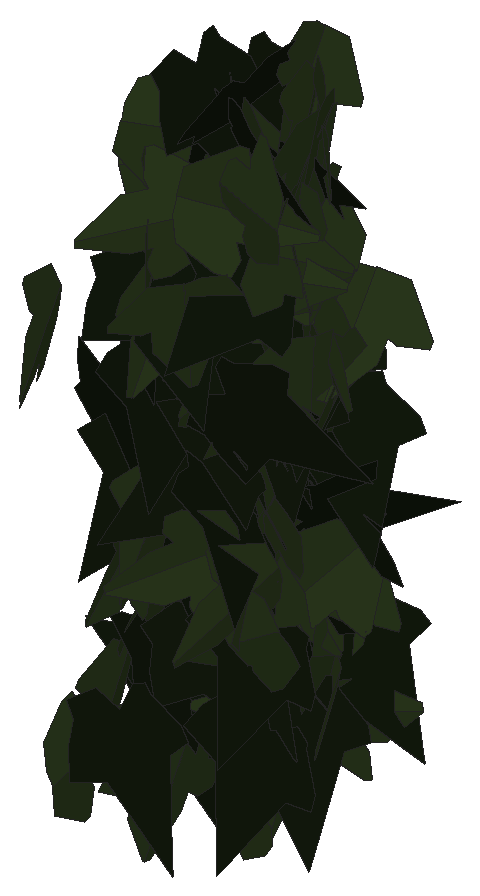
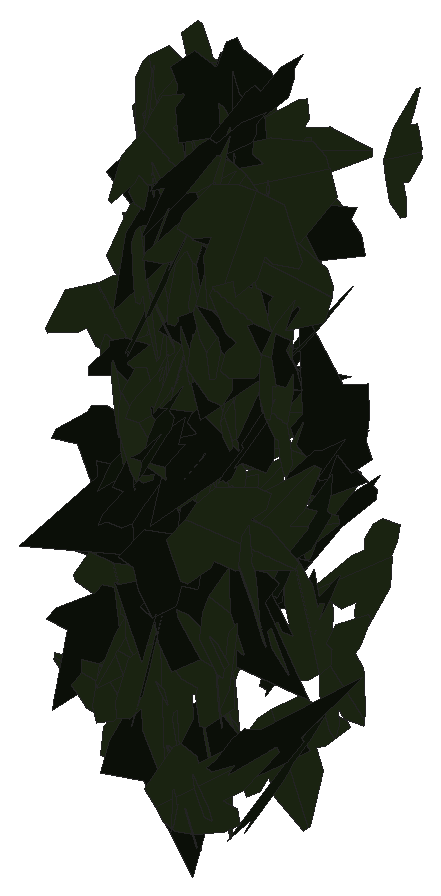
# SketchUp Ruby script. Lengths in inches.
U = 1.inch
M = Sketchup.active_model
def pt(a) = Geom::Point3d.new(a.map { |v| v * U })
def face(e, loops, mat)
  f = e.add_face(loops[0].map { |a| pt(a) })
  loops[1..].each { |l| e.add_face(l.map { |a| pt(a) }).erase! }
  f.material = f.back_material = mat if mat
  f
end
# faces: each face lists its corners as indices into pts; further lists are holes
def faces(e, pts, list, mat = nil) = list.each { |f| face(e, (f[0].is_a?(Array) ? f : [f]).map { |l| l.map { |i| pts[i] } }, mat) }
# xy, xz, yz: faces in a plane at the given z, y or x. An outline is a flat list of corners, or four numbers for a rectangle; further outlines are holes
def ring(l) = l.size == 4 ? [[l[0], l[1]], [l[2], l[1]], [l[2], l[3]], [l[0], l[3]]] : l.each_slice(2).to_a
def flat(e, list, mat, &to3) = list.each { |f| face(e, (f[0].is_a?(Array) ? f : [f]).map { |l| ring(l).map { |u, v| to3.(u, v) } }, mat) }
def xy(e, z, list, mat = nil) = flat(e, list, mat) { |x, y| [x, y, z] }
def xz(e, y, list, mat = nil) = flat(e, list, mat) { |x, z| [x, y, z] }
def yz(e, x, list, mat = nil) = flat(e, list, mat) { |y, z| [x, y, z] }
def lines(e, pts, list) = list.each { |a, b| e.add_line(pt(pts[a]), pt(pts[b])) }
# prism: a flat outline (further loops are holes) pulled along v
def prism(e, loops, v, mat = nil)
  f = face(e, loops, mat); d = Geom::Vector3d.new(v.map { |x| x * U })
  f.pushpull(f.normal.samedirection?(d) ? d.length : -d.length)
end
def box(e, o, s, mat = nil) = prism(e, [[o, [o[0] + s[0], o[1], o[2]], [o[0] + s[0], o[1] + s[1], o[2]], [o[0], o[1] + s[1], o[2]]]], [0, 0, s[2]], mat)
def at(x, y, z, deg = 0) = Geom::Transformation.translation(pt([x, y, z])) * Geom::Transformation.rotation(ORIGIN, Z_AXIS, deg.degrees)
def axes(o, x, y, z) = Geom::Transformation.new([*x, 0, *y, 0, *z, 0, *pt(o).to_a, 1])
def part(name) = M.definitions.add(name)
# library, detail: a bought-in or finely detailed component or shape, given as its bounding box
def library(name, o, s) = part(name).tap { |d| box(d.entities, o, s) }
def detail(e, o, s) = box(e.add_group.entities, o, s)
def put(e, d, t, mat = nil) = e.add_instance(d, t).tap { |i| i.material = mat if mat }
def group(e, t, mat = nil) = e.add_group.tap { |g| g.transformation = t; g.material = mat if mat }.entities
root = M.entities
M.materials.add("efeu1").color = [18, 25, 13]
M.materials.add("efeu2").color = [43, 57, 29]
c1 = part("ivyleaf_10")
p = [[0,0.5,-0.03],[-0.0625,2.02,-0.43],[-0.19,2.01,-0.46],[-0.54,1.05,-0.29],[-0.52,0.625,-0.18],[-0.83,0.76,-0.28],
  [-1.16,0.64,-0.33],[-1.15,0.33,-0.24],[-0.77,-0.39,0.02],[-0.3,-0.51,0.16],[0.04,-0.48,0.23],[-0.02,2.01,-0.4375],
  [-0.06,2.01,-0.43],[0.04,-0.49,0.23],[0.67,-0.49,0.14],[1.38,0.36,-0.2],[1.375,0.51,-0.24],[0.81,0.65,-0.19],
  [0.62,0.59,-0.15],[0.6,1.09,-0.28],[0.5,1.23,-0.31]]
faces(c1.entities,p,[[0,1,2,3,4,5,6,7,8,9,10],[11,12,0,13,14,15,16,17,18,19,20]],"efeu2")
c2 = part("ivyleaf_9")
p = [[1.54,2.16,1.25],[1.36,2.04,1.19],[-0.21,0.99,0.68],[-0.71,1.11,0.82],[-0.85,0.86,0.67],[-0.8,0.17,0.21],
  [-0.9,-0.01,0.1],[-0.67,-0.16,-0.02],[-0.08,-0.08,-0.05],[-0.03,-0.6,-0.4],[0.65,-0.88,-0.66],[0.83,-0.6,-0.49],
  [1.29,-0.42,-0.43],[1.8125,-0.07,-0.26],[1.21,0.44,0.15]]
faces(c2.entities,p,[[0,1,2,3,4,5,6,7,8,9,10,11,12,13,14]],"efeu1")
put(root,c1,axes([20.33,224.47,212.01],[0.02199,-0.25985,0.4266],[0.29049,-0.34074,-0.22253],[0.40637,0.25763,0.13598]))
put(root,c1,axes([20.39,224.75,209.6875],[0.27657,-0.28984,0.29917],[0.22612,-0.19712,-0.40001],[0.34983,0.35656,0.02204]))
put(root,c1,axes([20.49,223.3,208.03],[0.11424,-0.38823,0.29364],[0.15042,-0.25871,-0.40056],[0.46295,0.17986,0.05769]))
put(root,c1,axes([20.1875,224.12,212.7],[0.13224,-0.04593,-0.48],[0.48078,-0.02552,0.13489],[-0.03689,-0.49723,0.03742]))
put(root,c1,axes([20.26,224.33,211.28],[0.0721,-0.13957,0.47468],[0.43944,-0.20236,-0.12625],[0.22735,0.4354,0.09348]))
put(root,c2,axes([20.8,224.34,207.35],[-0.14741,-0.46669,-0.10235],[-0.0286,-0.0983,0.48941],[-0.47692,0.15014,0.00229]))
put(root,c2,axes([20.36,224.15,207.36],[0.28835,-0.40239,-0.07029],[-0.03998,0.05783,-0.49503],[0.40652,0.2911,0.00118]))
put(root,c1,axes([20.49,223.69,208.41],[0.10028,-0.48295,-0.08189],[0.04353,-0.07447,0.4925],[-0.4879,-0.10591,0.02711]))
put(root,c1,axes([20.61,224.31,212.125],[0.14595,-0.37319,0.29905],[-0.0825,0.28833,0.40008],[-0.47105,-0.16613,0.02259]))
put(root,c1,axes([20.68,224.44,213.45],[-0.47653,-0.11911,-0.09344],[0.09004,0.02512,-0.49118],[0.1217,-0.48496,-0.00249]))
put(root,c2,axes([20.5,223.28,210.45],[-0.14661,0.01383,0.47782],[0.27194,-0.40862,0.09526],[0.39313,0.28781,0.1123]))
put(root,c2,axes([20.75,223.64,210.09],[-0.168,-0.40585,0.23887],[-0.0897,-0.22139,-0.43925],[0.46231,-0.19044,0.00158]))
put(root,c1,axes([20.96,224.66,210.03],[0.23693,0.17825,-0.40261],[-0.32366,-0.23946,-0.29649],[-0.29851,0.40111,0.00191]))
put(root,c1,axes([20.97,224.02,209.59],[0.15587,0.39023,0.27097],[-0.14332,-0.23327,0.41838],[0.45295,-0.2081,0.03913]))
put(root,c1,axes([20.9375,224.51,212.03],[-0.10024,-0.25761,0.41664],[-0.05273,-0.41713,-0.2706],[0.487,-0.09819,0.05646]))
put(root,c1,axes([20.9,224.43,209.01],[-0.01172,-0.35546,0.35144],[0.01492,-0.35163,-0.35515],[0.49964,0.00216,0.01884]))
put(root,c2,axes([20.57,223.82,209.45],[0.13729,-0.38149,0.29261],[0.14125,-0.25887,-0.40377],[0.45957,0.19353,0.03669]))
put(root,c1,axes([21.2,223.97,209.51],[-0.10741,0.02729,-0.48756],[-0.44234,-0.21693,0.08531],[-0.20687,0.44967,0.07074]))
put(root,c1,axes([21.01,223.49,207.19],[-0.14845,-0.46369,0.11382],[-0.0205,-0.1129,-0.48666],[0.47701,-0.14916,0.01451]))
put(root,c2,axes([21.17,224.48,209.12],[0.06679,0.10665,-0.48391],[-0.23181,-0.42483,-0.12562],[-0.43795,0.24113,-0.0073]))
put(root,c2,axes([20.79,224.53,212.14],[-0.24225,-0.26612,-0.34713],[0.24778,0.24351,-0.35959],[0.36044,-0.34625,0.0139]))
put(root,c1,axes([20.67,223.5625,213.5],[-0.06645,-0.10428,-0.48447],[0.43348,0.22467,-0.10781],[0.24017,-0.43434,0.06055]))
put(root,c1,axes([21.2,224.76,206.98],[0.0638,0.22952,0.4396],[-0.17895,-0.40271,0.23623],[0.4625,-0.18748,0.03076]))
put(root,c1,axes([20.99,224.53,212.07],[-0.04955,-0.0893,-0.48946],[-0.01857,-0.49121,0.0915],[-0.49719,0.02724,0.04536]))
put(root,c2,axes([20.95,224.08,210.67],[-0.07109,-0.31814,0.37912],[-0.05505,-0.37555,-0.32547],[0.49185,-0.08802,0.01837]))
put(root,c1,axes([20.98,222.97,209.63],[-0.02382,0.17324,-0.46842],[-0.00525,-0.46902,-0.1732],[-0.4994,-0.00333,0.02417]))
put(root,c1,axes([20.83,224.6,208.26],[-0.19121,0.11981,0.44619],[0.38268,-0.22946,0.22561],[0.25883,0.42778,-0.00395]))
put(root,c2,axes([20.91,223.46,208.09],[-0.04585,-0.28402,0.40894],[0.08136,-0.40942,-0.27523],[0.4912,0.0413,0.08376]))
put(root,c1,axes([20.99,223.83,213.21],[-0.21145,0.39369,-0.22427],[0.11013,-0.19541,-0.44686],[-0.4395,-0.23838,-0.00408]))
put(root,c1,axes([21.18,222.91,213.125],[0.20495,-0.26203,-0.37328],[-0.0615,0.38962,-0.30727],[0.4519,0.17186,0.12747]))
put(root,c1,axes([21.43,223.83,209.91],[-0.25121,0.0809,0.42467],[-0.40099,0.13995,-0.26386],[-0.16156,-0.47315,-0.00543]))
put(root,c2,axes([21.36,224.57,209.7],[0.04944,0.09554,-0.48829],[-0.18944,-0.45012,-0.10725],[-0.46008,0.1956,-0.00831]))
put(root,c1,axes([21.43,223.8,209.47],[-0.40038,0.04799,-0.29562],[-0.29401,0.03099,0.40323],[0.05703,0.49673,0.0034]))
put(root,c2,axes([20.83,224.18,212.09],[-0.00282,0.0064,0.49995],[0.44408,-0.2297,0.00544],[0.22974,0.44407,-0.00439]))
put(root,c1,axes([21.11,223.04,210.05],[-0.00707,-0.27112,0.42006],[0.24254,-0.36921,-0.23422],[0.43718,0.20045,0.13674]))
put(root,c1,axes([21.32,223.82,211.64],[-0.08835,-0.48831,-0.06125],[0.00843,0.06072,-0.49623],[0.49206,-0.08872,-0.0025]))
put(root,c1,axes([21.16,224.08,213.38],[-0.44404,0.06872,-0.21933],[0.2115,-0.06462,-0.44843],[-0.08998,-0.49102,0.02832]))
put(root,c1,axes([20.93,224.62,208.43],[-0.05053,-0.03477,-0.49622],[0.43774,-0.24003,-0.02776],[-0.23628,-0.43724,0.05469]))
put(root,c1,axes([21.12,221.56,212.65],[0.05843,-0.18373,0.46134],[0.28071,-0.37096,-0.18328],[0.40962,0.28042,0.0598]))
put(root,c1,axes([21.32,223.07,212.28],[0.16206,0.40936,-0.23699],[-0.1132,-0.20967,-0.43957],[-0.45926,0.19613,0.02472]))
put(root,c2,axes([21.13,223.15,211.19],[0.01142,-0.43871,0.23959],[0.06062,-0.23666,-0.43625],[0.49618,0.03901,0.04778]))
put(root,c1,axes([21.21,223.91,210.91],[-0.0944,0.07581,0.48512],[0.23342,-0.42768,0.11225],[0.43198,0.24767,0.04535]))
put(root,c1,axes([21.33,221.55,208.11],[0.03324,0.06885,-0.49412],[0.09879,0.4845,0.07415],[0.48902,-0.10256,0.01861]))
put(root,c2,axes([21.21,223.57,214.21],[0.1947,-0.3798,-0.26047],[-0.12035,0.23101,-0.42679],[0.44453,0.22889,-0.00146]))
put(root,c1,axes([21.57,222.95,213.16],[-0.08204,0.00789,0.49316],[-0.19676,-0.45896,-0.02539],[0.45228,-0.19823,0.07841]))
put(root,c1,axes([21.4,224.3,212.46],[0.018,-0.48347,-0.12621],[0.01884,0.12686,-0.48327],[0.49932,0.01264,0.02278]))
put(root,c1,axes([21.39,224.14,212.15],[0.1284,-0.47979,0.05762],[0.02117,-0.05398,-0.49663],[0.48277,0.12997,0.00645]))
put(root,c1,axes([21.45,223.97,207.24],[0.21759,-0.44661,-0.05649],[-0.02036,0.05291,-0.49678],[0.44971,0.21849,0.00484]))
put(root,c2,axes([21.29,222.94,212.49],[-0.12408,-0.37575,-0.30564],[0.07552,0.29664,-0.39535],[0.47844,-0.14427,-0.01686]))
put(root,c1,axes([21.66,224.17,207.12],[-0.08736,0.11992,0.47748],[-0.34063,0.3354,-0.14656],[-0.35544,-0.3509,0.02309]))
put(root,c2,axes([21.25,224.2,213.9],[0.17784,-0.39563,-0.2487],[-0.0334,0.25466,-0.42899],[0.46611,0.1692,0.06416]))
put(root,c2,axes([21.57,224.35,207.49],[0.09853,0.45706,-0.17716],[-0.03713,-0.17322,-0.46756],[-0.48879,0.1053,-0.0002]))
put(root,c2,axes([21.33,223.76,210.89],[0.45031,0.21473,-0.0334],[-0.03092,-0.01276,-0.49888],[-0.2151,0.45136,0.00179]))
put(root,c1,axes([21.56,223.55,208.05],[0.17449,-0.23474,0.40552],[-0.2083,0.34876,0.29151],[-0.41972,-0.27068,0.02391]))
put(root,c1,axes([21.32,223.82,208.77],[-0.35218,-0.14555,-0.32371],[0.2951,0.13329,-0.38099],[0.1972,-0.4594,-0.00798]))
put(root,c1,axes([21.43,224.12,212.88],[0.05489,0.47909,0.13214],[-0.00338,0.1333,-0.48189],[-0.49697,0.05201,0.01787]))
put(root,c1,axes([21.47,223.88,213.79],[-0.36924,0.3338,-0.0473],[0.03223,-0.03488,-0.49774],[-0.33559,-0.37062,0.00424]))
put(root,c2,axes([21.08,223.88,208.67],[0.28543,-0.03112,0.40934],[0.40576,-0.05439,-0.28706],[0.06239,0.49606,-0.00579]))
put(root,c1,axes([21.48,224.48,207.15],[0.4165,-0.2726,0.04709],[0.03821,-0.0276,-0.49777],[0.27398,0.41824,-0.00216]))
put(root,c2,axes([21.37,223.52,211.91],[-0.08254,-0.431,-0.23964],[0.08926,0.2259,-0.43704],[0.48499,-0.11493,0.03965]))
put(root,c2,axes([21.73,223.53,214.25],[-0.16223,0.42894,-0.19923],[0.06301,-0.18914,-0.45854],[-0.46873,-0.17388,0.00731]))
put(root,c1,axes([21.66,224.49,208.125],[-0.17755,-0.46618,-0.03402],[0.01349,0.03126,-0.49884],[0.46722,-0.17805,0.00147]))
put(root,c2,axes([21.41,224.11,211.21],[0.2357,-0.43849,-0.04656],[-0.02285,0.04058,-0.49783],[0.44037,0.2368,-0.00091]))
put(root,c1,axes([21.77,223.5625,206.96],[0.02568,-0.0329,0.49826],[-0.25136,0.43024,0.04136],[-0.43146,-0.25261,0.00556]))
put(root,c2,axes([21.76,223.25,210.6],[-0.27789,-0.28502,0.30256],[-0.16684,-0.25686,-0.39521],[0.38071,-0.3206,0.04765]))
put(root,c2,axes([21.49,224.92,212.3],[0.01058,-0.29028,0.40697],[0.02076,-0.40646,-0.29045],[0.49946,0.02304,0.00345]))
put(root,c2,axes([21.38,223.7,209.05],[0.45745,-0.2018,0.00432],[0.00602,0.00295,-0.49996],[0.20176,0.45746,0.00512]))
put(root,c1,axes([21.58,224.23,211.64],[-0.09819,0.4213,-0.25072],[0.05489,-0.24465,-0.43259],[-0.48718,-0.11248,0.00179]))
put(root,c2,axes([21.47,223.43,208.83],[-0.00097,-0.34128,-0.36541],[0.09696,0.35835,-0.33494],[0.49051,-0.07151,0.06549]))
put(root,c1,axes([21.97,224.2,211.82],[0.15486,0.01745,0.47509],[-0.4197,0.23973,0.128],[-0.22332,-0.43844,0.0889]))
put(root,c1,axes([21.69,224.66,214.06],[0.05988,0.38804,-0.30958],[-0.05549,-0.30464,-0.39258],[-0.49329,0.08137,0.00658]))
put(root,c1,axes([21.54,224.3,211.48],[0.42074,0.22166,0.15442],[0.12976,0.08487,-0.47535],[-0.23694,0.44007,0.01389]))
put(root,c2,axes([21.58,224.88,208.17],[-0.00172,-0.11602,0.48635],[0.01387,-0.48618,-0.11593],[0.4998,0.01309,0.00489]))
put(root,c2,axes([21.54,223.67,210.41],[0.16884,-0.47063,0.00032],[0.00007,-0.00032,-0.5],[0.47063,0.16884,-0.00004]))
put(root,c1,axes([21.65,223.37,210.16],[-0.04641,-0.26349,0.42239],[0.07248,0.41613,0.26755],[-0.49254,0.08607,-0.00043]))
put(root,c1,axes([21.76,223.58,207.82],[0.24687,-0.42493,0.09213],[0.0384,-0.08422,-0.49136],[0.43311,0.24967,-0.00895]))
put(root,c1,axes([21.62,223.96,210.94],[0.4457,-0.15396,0.16627],[0.15828,-0.05103,-0.47153],[0.16216,0.47296,0.00324]))
put(root,c2,axes([21.83,224.8,210.1875],[-0.14033,-0.28072,0.38924],[-0.18827,-0.34083,-0.31368],[0.44143,-0.23459,-0.01005]))
put(root,c1,axes([21.84,222.59,212.54],[-0.30874,-0.39135,-0.03903],[0.02026,0.03372,-0.49845],[0.39277,-0.30937,-0.00496]))
put(root,c1,axes([21.98,223.65,213.28],[-0.45518,-0.09163,0.18551],[-0.17623,-0.06318,-0.46363],[0.1084,-0.48746,0.02522]))
put(root,c1,axes([21.88,224.44,212.61],[0.11893,-0.47014,-0.12177],[-0.03791,0.116,-0.48488],[0.48417,0.12457,-0.00806]))
put(root,c1,axes([21.79,224.74,211.04],[0.13508,-0.42202,0.23163],[0.08623,-0.21547,-0.44287],[0.47362,0.15959,0.01457]))
put(root,c1,axes([21.75,223.75,209.49],[-0.20318,0.39766,-0.2249],[0.10087,-0.20102,-0.44656],[-0.44558,-0.22684,0.00146]))
put(root,c1,axes([21.78,224.69,210.82],[-0.03083,-0.12085,0.48419],[0.17711,-0.45619,-0.10259],[0.46656,0.16519,0.07093]))
put(root,c1,axes([22.12,223.48,210.16],[-0.3668,0.13238,0.31294],[-0.31418,0.04327,-0.38655],[-0.12943,-0.48021,0.05144]))
put(root,c2,axes([21.74,223.92,211.09],[-0.1305,-0.44055,-0.1972],[0.06064,0.1877,-0.45945],[0.47885,-0.14383,0.00444]))
put(root,c2,axes([21.77,224.04,213.32],[0.46761,0.10339,-0.14369],[-0.13999,-0.03245,-0.47891],[-0.10836,0.48812,-0.0014]))
put(root,c1,axes([22.09,222.68,210.05],[0.086,0.08182,-0.48571],[-0.3418,-0.3451,-0.11865],[-0.35465,0.35243,-0.00343]))
put(root,c2,axes([21.65,224.45,210.9375],[0.38808,-0.3076,-0.06909],[-0.0545,0.04247,-0.4952],[0.31052,0.39189,-0.00057]))
put(root,c2,axes([21.7,221.87,208.625],[0.13677,-0.46034,-0.1392],[-0.02262,0.13841,-0.47993],[0.4804,0.13757,0.01703]))
put(root,c2,axes([21.83,224.42,211.59],[-0.23766,-0.41491,-0.14618],[0.07689,0.12441,-0.47813],[0.43313,-0.24974,0.00467]))
put(root,c1,axes([21.91,223.69,209.91],[0.05095,-0.3791,-0.322],[0.0731,0.32588,-0.3721],[0.492,-0.00916,0.08864]))
put(root,c2,axes([22.04,224.38,209.71],[0.32552,0.15583,-0.34605],[-0.31527,-0.14278,-0.36086],[-0.21128,0.45314,0.0053]))
put(root,c1,axes([22.09,224.26,207.89],[-0.28001,-0.40037,0.1063],[-0.05656,-0.09016,-0.48854],[0.41036,-0.28562,0.0052]))
put(root,c2,axes([21.6,223.61,213.7],[0.21481,0.0105,-0.45138],[0.45124,0.01207,0.21502],[0.01541,-0.49974,-0.00429]))
put(root,c1,axes([21.88,224.24,213.83],[0.12328,-0.29242,0.38639],[0.25836,-0.29763,-0.30768],[0.40994,0.27551,0.07771]))
put(root,c2,axes([22.0625,223.34,212.58],[-0.20613,-0.36224,0.27621],[-0.07563,-0.27175,-0.41284],[0.44921,-0.21197,0.05724]))
put(root,c1,axes([22.02,223.83,213.03],[-0.2467,0.43197,-0.05044],[0.02156,-0.04577,-0.49743],[-0.43437,-0.24761,0.00396]))
put(root,c1,axes([22.12,224.52,211.12],[0.17501,-0.46007,-0.0878],[-0.0204,0.08616,-0.4921],[0.46793,0.17582,0.01138]))
put(root,c1,axes([21.73,223.4375,212.45],[-0.00565,-0.05492,-0.49694],[0.49622,0.06015,-0.01229],[0.06114,-0.49332,0.05382]))
put(root,c1,axes([22.07,224.59,209],[0.49936,-0.00572,-0.02458],[-0.02452,0.005,-0.49937],[0.00596,0.49994,0.00471]))
put(root,c1,axes([22.09,223.85,209.3125],[-0.02695,0.44355,0.22922],[-0.04246,0.22668,-0.44364],[-0.49746,-0.04338,0.02545]))
put(root,c1,axes([22.26,224.27,209.33],[0.18448,0.20643,-0.41636],[-0.26358,-0.32246,-0.27667],[-0.38274,0.32157,-0.01015]))
put(root,c1,axes([22.5,222.85,209.3],[-0.2357,-0.06959,0.43543],[-0.42235,-0.1063,-0.24561],[0.12675,-0.48359,-0.00867]))
put(root,c1,axes([22.22,223.91,211.56],[-0.27402,-0.4182,-0.00493],[0.00308,0.00387,-0.49998],[0.41822,-0.27404,0.00046]))
put(root,c1,axes([22.17,224.08,208.46],[0.0027,-0.22677,-0.44561],[0.04951,0.44355,-0.22542],[0.49753,-0.04291,0.02485]))
put(root,c1,axes([21.84,222.87,213.36],[0.05814,0.06632,0.49216],[0.35724,0.33862,-0.08783],[-0.34496,0.36185,-0.00801]))
put(root,c1,axes([21.99,224.16,211.9],[-0.34185,0.22168,-0.28981],[0.22344,-0.18677,-0.40643],[-0.28846,-0.4074,0.02863]))
put(root,c1,axes([22.21,224.17,212.35],[0.02143,0.26826,0.4214],[-0.00208,-0.42173,0.26858],[0.49954,-0.01326,-0.01696]))
put(root,c2,axes([22.09,223.43,207.89],[-0.09938,-0.45964,0.16986],[-0.03016,-0.16726,-0.47023],[0.4891,-0.10371,0.00552]))
put(root,c1,axes([22.22,224.11,208.12],[0.31159,-0.38029,-0.09106],[-0.05655,0.07138,-0.49164],[0.38693,0.31667,0.00147]))
put(root,c2,axes([22.08,223.83,208.02],[-0.10785,-0.4521,-0.18432],[0.03141,0.18195,-0.46466],[0.48722,-0.11181,-0.01085]))
put(root,c2,axes([21.96,223.05,210.29],[0.05776,-0.41879,0.26698],[0.10108,-0.25324,-0.41911],[0.48626,0.10239,0.05541]))
put(root,c2,axes([22.05,224.53,210.73],[-0.1661,-0.38065,-0.27841],[0.14473,0.23979,-0.41419],[0.44885,-0.21818,0.03053]))
put(root,c1,axes([22.17,223.75,213.05],[0.14695,-0.45646,0.1416],[-0.04388,0.13463,0.47953],[-0.4759,-0.15336,-0.00049]))
put(root,c2,axes([22,224.13,209.72],[0.27785,0.20189,0.36338],[0.28187,0.22974,-0.34317],[-0.30553,0.39555,0.01385]))
put(root,c1,axes([21.95,224.34,213.81],[0.12541,-0.17066,0.45293],[0.3885,-0.24358,-0.19934],[0.28869,0.40193,0.07151]))
put(root,c1,axes([22.625,222.74,213.59],[0.03474,0.02033,0.49838],[-0.49633,0.051,0.03252],[-0.04952,-0.49698,0.02372]))
put(root,c1,axes([21.89,224.52,207.61],[0.12369,-0.00247,-0.48445],[0.4815,-0.05453,0.12321],[-0.05344,-0.49701,-0.01111]))
put(root,c2,axes([22.21,223.29,209.02],[-0.09704,-0.45228,0.18981],[-0.01887,-0.1899,-0.46215],[0.49013,-0.09685,0.01979]))
put(root,c1,axes([22.36,222.91,209.72],[-0.02167,-0.20172,0.45699],[0.0214,-0.45738,-0.20087],[0.49907,0.01086,0.02846]))
put(root,c2,axes([22.13,224.4375,208.58],[-0.06041,-0.29516,-0.39904],[0.10393,0.38555,-0.30091],[0.48533,-0.1193,0.01477]))
put(root,c1,axes([22.2,223.33,212.82],[0.04017,-0.27089,-0.41833],[0.21219,0.38905,-0.23155],[0.45095,-0.15893,0.14622]))
put(root,c2,axes([21.96,223.09,211.375],[0.08325,0.04572,-0.4909],[0.36122,0.33317,0.09229],[0.33555,-0.37001,0.02244]))
put(root,c1,axes([22.38,223.68,213.99],[0.06606,-0.49413,-0.0384],[0.00094,0.03886,-0.49849],[0.49562,0.06579,0.00606]))
put(root,c1,axes([22.37,224.45,211.96],[0.37489,0.28826,-0.16237],[-0.12605,-0.10243,-0.47288],[-0.30589,0.39549,-0.00413]))
